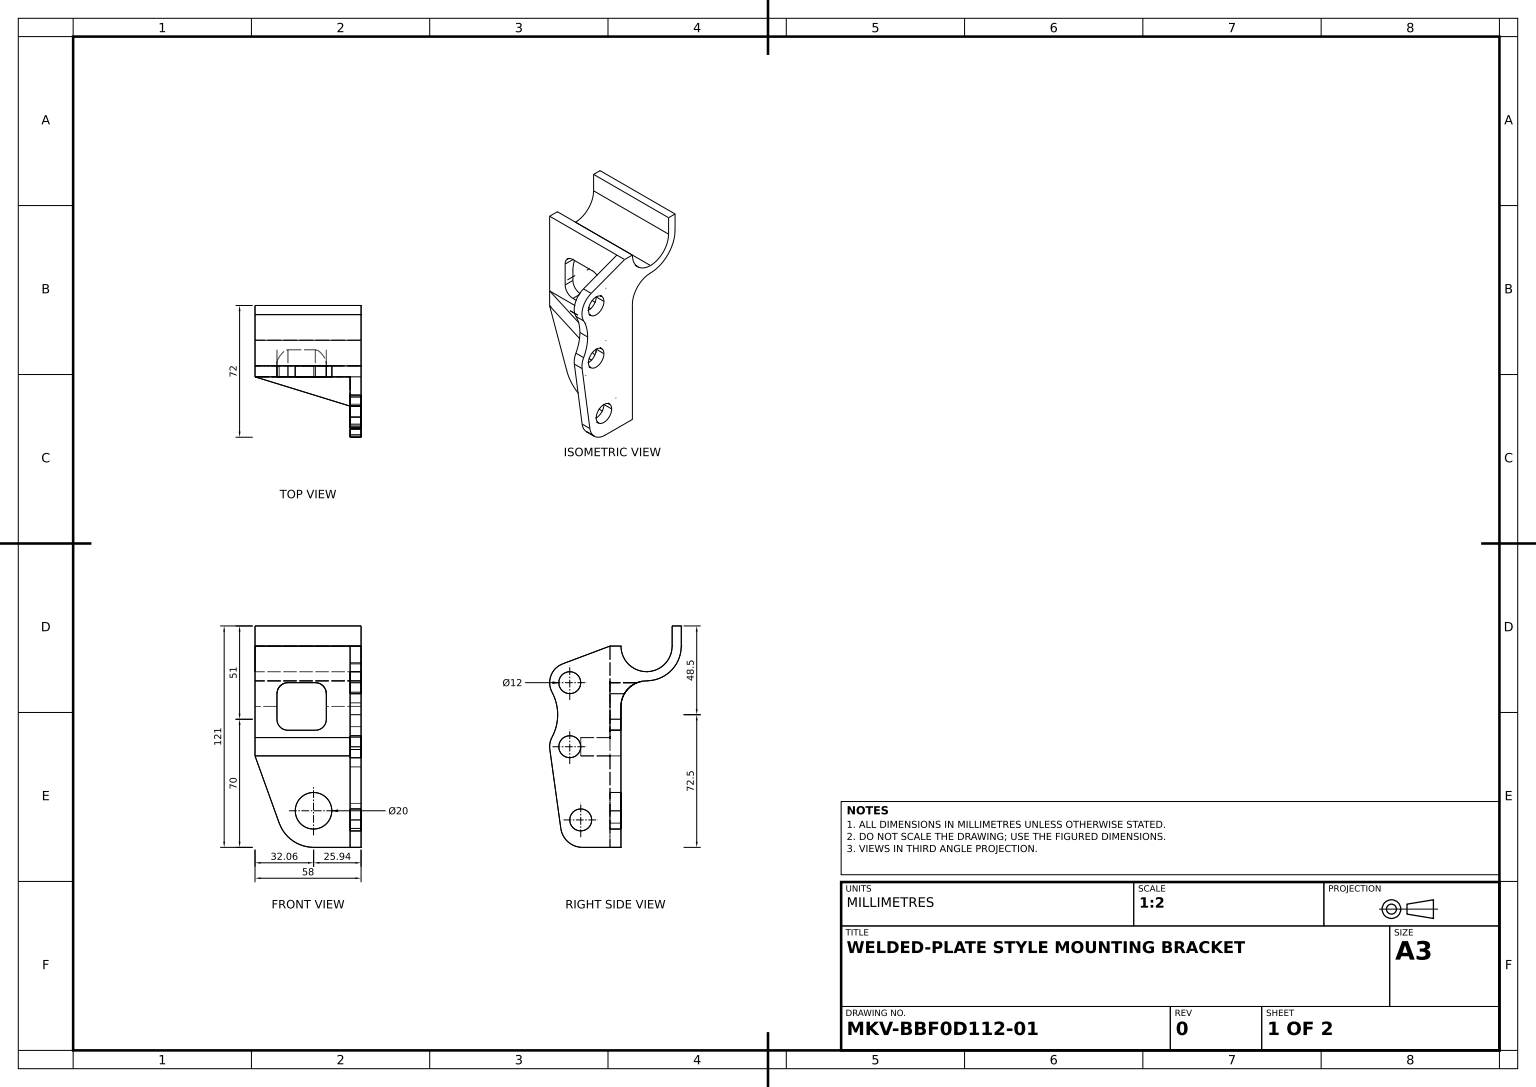
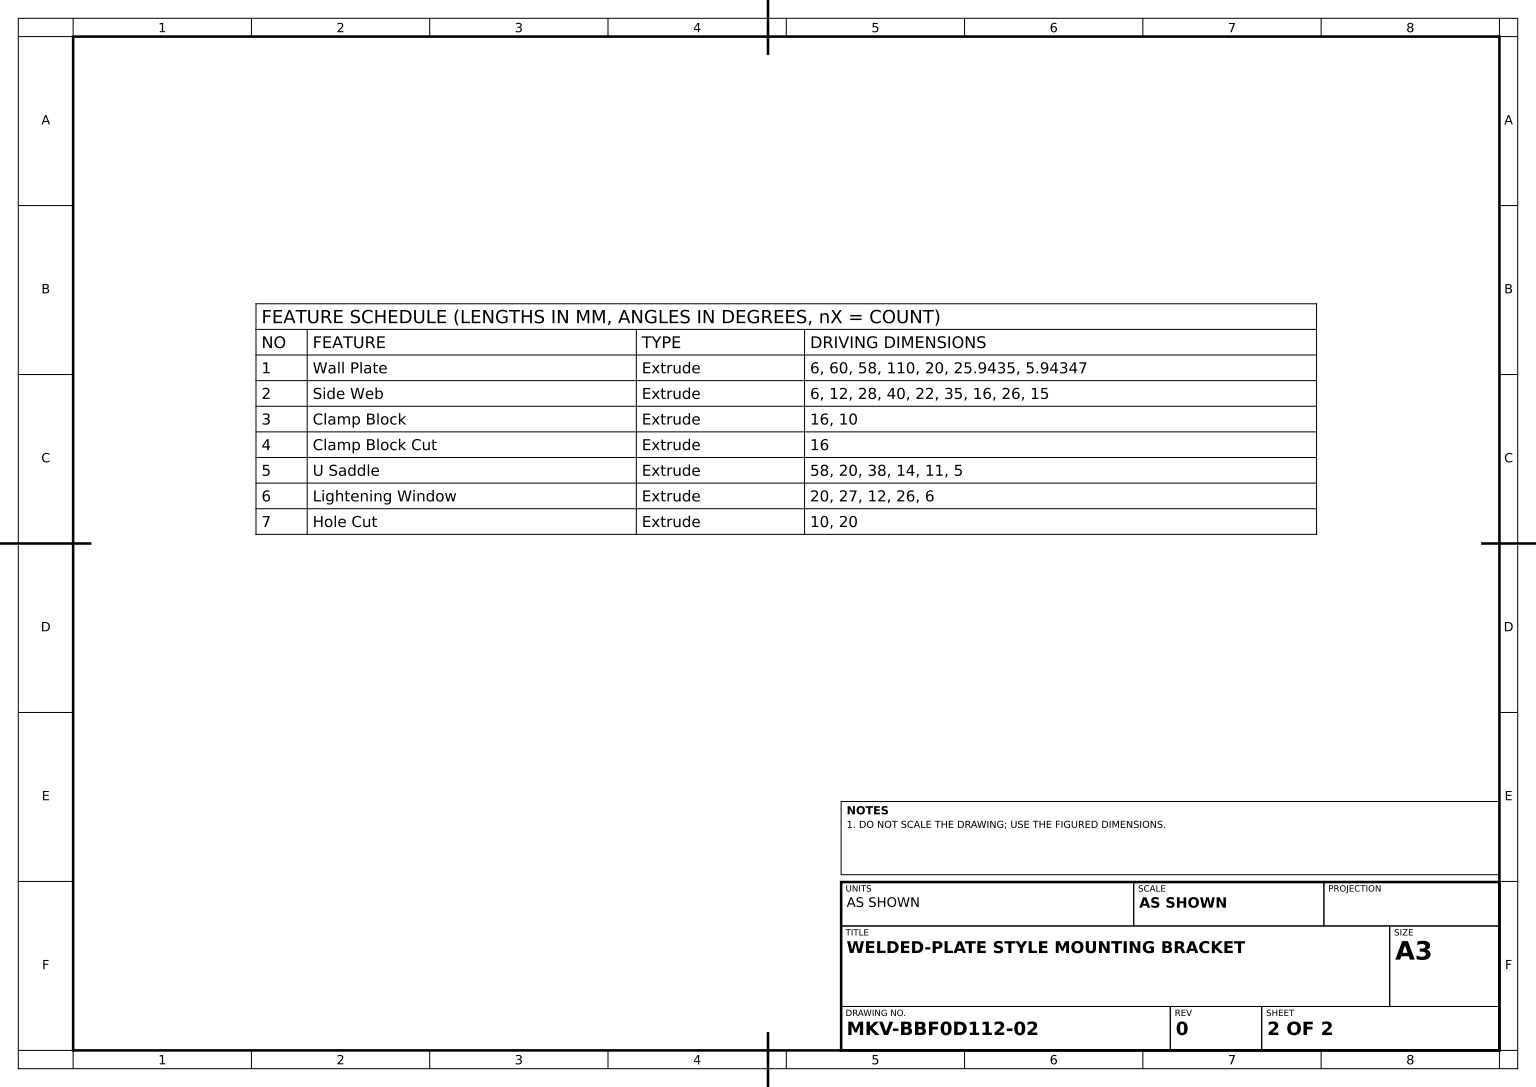
ISO-10303-21;
HEADER;
FILE_DESCRIPTION((''),'2;1');
FILE_NAME('','',(''),(''),'','','');
FILE_SCHEMA(('AUTOMOTIVE_DESIGN'));
ENDSEC;
DATA;
#1=APPLICATION_CONTEXT('');
#2=PRODUCT_CONTEXT('',#1,'mechanical');
#3=PRODUCT('','','',(#2));
#4=PRODUCT_DEFINITION_FORMATION('','',#3);
#5=PRODUCT_DEFINITION_CONTEXT('',#1,'design');
#6=PRODUCT_DEFINITION('','',#4,#5);
#7=PRODUCT_DEFINITION_SHAPE('','',#6);
#8=(LENGTH_UNIT()NAMED_UNIT(*)SI_UNIT(.MILLI.,.METRE.));
#9=(NAMED_UNIT(*)PLANE_ANGLE_UNIT()SI_UNIT($,.RADIAN.));
#10=(NAMED_UNIT(*)SI_UNIT($,.STERADIAN.)SOLID_ANGLE_UNIT());
#11=UNCERTAINTY_MEASURE_WITH_UNIT(LENGTH_MEASURE(1.E-05),#8,'distance_accuracy_value','');
#12=(GEOMETRIC_REPRESENTATION_CONTEXT(3)GLOBAL_UNCERTAINTY_ASSIGNED_CONTEXT((#11))GLOBAL_UNIT_ASSIGNED_CONTEXT((#8,#9,#10))REPRESENTATION_CONTEXT('',''));
#13=CARTESIAN_POINT('',(52.,0.,6.));
#14=VERTEX_POINT('',#13);
#15=CARTESIAN_POINT('',(0.,0.,6.));
#16=VERTEX_POINT('',#15);
#17=DIRECTION('',(-1.,0.,0.));
#18=VECTOR('',#17,1000.);
#19=LINE('',#15,#18);
#20=EDGE_CURVE('',#14,#16,#19,.T.);
#21=ORIENTED_EDGE('',*,*,#20,.F.);
#22=CARTESIAN_POINT('',(58.,0.,6.));
#23=VERTEX_POINT('',#22);
#24=EDGE_CURVE('',#23,#14,#19,.T.);
#25=ORIENTED_EDGE('',*,*,#24,.F.);
#26=CARTESIAN_POINT('',(58.,0.,0.));
#27=VERTEX_POINT('',#26);
#28=DIRECTION('',(0.,0.,-1.));
#29=VECTOR('',#28,1000.);
#30=LINE('',#22,#29);
#31=EDGE_CURVE('',#23,#27,#30,.T.);
#32=ORIENTED_EDGE('',*,*,#31,.T.);
#33=CARTESIAN_POINT('',(0.,0.,0.));
#34=VERTEX_POINT('',#33);
#35=LINE('',#33,#18);
#36=EDGE_CURVE('',#27,#34,#35,.T.);
#37=ORIENTED_EDGE('',*,*,#36,.T.);
#38=LINE('',#15,#29);
#39=EDGE_CURVE('',#16,#34,#38,.T.);
#40=ORIENTED_EDGE('',*,*,#39,.F.);
#41=EDGE_LOOP('',(#21,#25,#32,#37,#40));
#42=FACE_OUTER_BOUND('',#41,.T.);
#43=DIRECTION('',(0.,-1.,0.));
#44=AXIS2_PLACEMENT_3D('',#15,#43,#28);
#45=PLANE('',#44);
#46=ADVANCED_FACE('',(#42),#45,.F.);
#47=CARTESIAN_POINT('',(52.,-95.,16.));
#48=VERTEX_POINT('',#47);
#49=CARTESIAN_POINT('',(58.,-95.,16.));
#50=VERTEX_POINT('',#49);
#51=DIRECTION('',(1.,0.,0.));
#52=VECTOR('',#51,1000.);
#53=LINE('',#47,#52);
#54=EDGE_CURVE('',#48,#50,#53,.T.);
#55=ORIENTED_EDGE('',*,*,#54,.F.);
#56=CARTESIAN_POINT('',(52.,-95.,28.));
#57=VERTEX_POINT('',#56);
#58=CARTESIAN_POINT('',(52.,-95.,22.));
#59=AXIS2_PLACEMENT_3D('',#58,#51,#28);
#60=CIRCLE('',#59,6.);
#61=EDGE_CURVE('',#57,#48,#60,.T.);
#62=ORIENTED_EDGE('',*,*,#61,.F.);
#63=CARTESIAN_POINT('',(58.,-95.,28.));
#64=VERTEX_POINT('',#63);
#65=LINE('',#56,#52);
#66=EDGE_CURVE('',#57,#64,#65,.T.);
#67=ORIENTED_EDGE('',*,*,#66,.T.);
#68=CARTESIAN_POINT('',(58.,-95.,22.));
#69=AXIS2_PLACEMENT_3D('',#68,#51,#28);
#70=CIRCLE('',#69,6.);
#71=EDGE_CURVE('',#64,#50,#70,.T.);
#72=ORIENTED_EDGE('',*,*,#71,.T.);
#73=EDGE_LOOP('',(#55,#62,#67,#72));
#74=FACE_OUTER_BOUND('',#73,.T.);
#75=CYLINDRICAL_SURFACE('',#59,6.);
#76=ADVANCED_FACE('',(#74),#75,.F.);
#77=CARTESIAN_POINT('',(58.,11.,-33.));
#78=VERTEX_POINT('',#77);
#79=CARTESIAN_POINT('',(0.,11.,-33.));
#80=VERTEX_POINT('',#79);
#81=LINE('',#77,#18);
#82=EDGE_CURVE('',#78,#80,#81,.T.);
#83=ORIENTED_EDGE('',*,*,#82,.F.);
#84=CARTESIAN_POINT('',(58.,0.,-33.));
#85=VERTEX_POINT('',#84);
#86=DIRECTION('',(0.,1.,0.));
#87=VECTOR('',#86,1000.);
#88=LINE('',#84,#87);
#89=EDGE_CURVE('',#85,#78,#88,.T.);
#90=ORIENTED_EDGE('',*,*,#89,.F.);
#91=CARTESIAN_POINT('',(0.,0.,-33.));
#92=VERTEX_POINT('',#91);
#93=LINE('',#84,#18);
#94=EDGE_CURVE('',#85,#92,#93,.T.);
#95=ORIENTED_EDGE('',*,*,#94,.T.);
#96=LINE('',#91,#87);
#97=EDGE_CURVE('',#92,#80,#96,.T.);
#98=ORIENTED_EDGE('',*,*,#97,.T.);
#99=EDGE_LOOP('',(#83,#90,#95,#98));
#100=FACE_OUTER_BOUND('',#99,.T.);
#101=DIRECTION('',(0.,0.,1.));
#102=AXIS2_PLACEMENT_3D('',#84,#101,#51);
#103=PLANE('',#102);
#104=ADVANCED_FACE('',(#100),#103,.F.);
#105=CARTESIAN_POINT('',(22.,-90.,0.));
#106=VERTEX_POINT('',#105);
#107=CARTESIAN_POINT('',(22.,-90.,6.));
#108=VERTEX_POINT('',#107);
#109=CARTESIAN_POINT('',(22.,-90.,-4.));
#110=VECTOR('',#101,1000.);
#111=LINE('',#109,#110);
#112=EDGE_CURVE('',#106,#108,#111,.T.);
#113=ORIENTED_EDGE('',*,*,#112,.F.);
#114=CARTESIAN_POINT('',(42.,-90.,0.));
#115=VERTEX_POINT('',#114);
#116=CARTESIAN_POINT('',(32.,-90.,0.));
#117=AXIS2_PLACEMENT_3D('',#116,#28,#17);
#118=CIRCLE('',#117,10.);
#119=EDGE_CURVE('',#106,#115,#118,.T.);
#120=ORIENTED_EDGE('',*,*,#119,.T.);
#121=CARTESIAN_POINT('',(42.,-90.,6.));
#122=VERTEX_POINT('',#121);
#123=CARTESIAN_POINT('',(42.,-90.,-4.));
#124=LINE('',#123,#110);
#125=EDGE_CURVE('',#115,#122,#124,.T.);
#126=ORIENTED_EDGE('',*,*,#125,.T.);
#127=CARTESIAN_POINT('',(32.,-90.,6.));
#128=AXIS2_PLACEMENT_3D('',#127,#101,#51);
#129=CIRCLE('',#128,10.);
#130=EDGE_CURVE('',#122,#108,#129,.T.);
#131=ORIENTED_EDGE('',*,*,#130,.T.);
#132=EDGE_LOOP('',(#113,#120,#126,#131));
#133=FACE_OUTER_BOUND('',#132,.T.);
#134=CARTESIAN_POINT('',(32.,-90.,-4.));
#135=AXIS2_PLACEMENT_3D('',#134,#101,#51);
#136=CYLINDRICAL_SURFACE('',#135,10.);
#137=ADVANCED_FACE('',(#133),#136,.F.);
#138=EDGE_CURVE('',#48,#57,#60,.T.);
#139=ORIENTED_EDGE('',*,*,#138,.F.);
#140=ORIENTED_EDGE('',*,*,#54,.T.);
#141=EDGE_CURVE('',#50,#64,#70,.T.);
#142=ORIENTED_EDGE('',*,*,#141,.T.);
#143=ORIENTED_EDGE('',*,*,#66,.F.);
#144=EDGE_LOOP('',(#139,#140,#142,#143));
#145=FACE_OUTER_BOUND('',#144,.T.);
#146=ADVANCED_FACE('',(#145),#75,.F.);
#147=CARTESIAN_POINT('',(58.,-20.,22.));
#148=VERTEX_POINT('',#147);
#149=CARTESIAN_POINT('',(58.,-20.,34.));
#150=VERTEX_POINT('',#149);
#151=CARTESIAN_POINT('',(58.,-20.,28.));
#152=AXIS2_PLACEMENT_3D('',#151,#51,#28);
#153=CIRCLE('',#152,6.);
#154=EDGE_CURVE('',#148,#150,#153,.T.);
#155=ORIENTED_EDGE('',*,*,#154,.T.);
#156=CARTESIAN_POINT('',(52.,-20.,34.));
#157=VERTEX_POINT('',#156);
#158=LINE('',#156,#52);
#159=EDGE_CURVE('',#157,#150,#158,.T.);
#160=ORIENTED_EDGE('',*,*,#159,.F.);
#161=CARTESIAN_POINT('',(52.,-20.,22.));
#162=VERTEX_POINT('',#161);
#163=CARTESIAN_POINT('',(52.,-20.,28.));
#164=AXIS2_PLACEMENT_3D('',#163,#51,#28);
#165=CIRCLE('',#164,6.);
#166=EDGE_CURVE('',#162,#157,#165,.T.);
#167=ORIENTED_EDGE('',*,*,#166,.F.);
#168=LINE('',#161,#52);
#169=EDGE_CURVE('',#162,#148,#168,.T.);
#170=ORIENTED_EDGE('',*,*,#169,.T.);
#171=EDGE_LOOP('',(#155,#160,#167,#170));
#172=FACE_OUTER_BOUND('',#171,.T.);
#173=CYLINDRICAL_SURFACE('',#164,6.);
#174=ADVANCED_FACE('',(#172),#173,.F.);
#175=CARTESIAN_POINT('',(12.,-26.,-1.875644));
#176=VERTEX_POINT('',#175);
#177=CARTESIAN_POINT('',(12.,-26.,6.));
#178=VERTEX_POINT('',#177);
#179=CARTESIAN_POINT('',(12.,-26.,-14.));
#180=LINE('',#179,#110);
#181=EDGE_CURVE('',#176,#178,#180,.T.);
#182=ORIENTED_EDGE('',*,*,#181,.T.);
#183=CARTESIAN_POINT('',(12.,-40.,6.));
#184=VERTEX_POINT('',#183);
#185=VECTOR('',#43,1000.);
#186=LINE('',#177,#185);
#187=EDGE_CURVE('',#178,#184,#186,.T.);
#188=ORIENTED_EDGE('',*,*,#187,.T.);
#189=CARTESIAN_POINT('',(12.,-40.,0.));
#190=VERTEX_POINT('',#189);
#191=CARTESIAN_POINT('',(12.,-40.,-14.));
#192=LINE('',#191,#110);
#193=EDGE_CURVE('',#190,#184,#192,.T.);
#194=ORIENTED_EDGE('',*,*,#193,.F.);
#195=CARTESIAN_POINT('',(12.,-33.,0.));
#196=VERTEX_POINT('',#195);
#197=CARTESIAN_POINT('',(12.,-90.,0.));
#198=LINE('',#197,#87);
#199=EDGE_CURVE('',#190,#196,#198,.T.);
#200=ORIENTED_EDGE('',*,*,#199,.T.);
#201=CARTESIAN_POINT('',(12.,-33.,-14.));
#202=AXIS2_PLACEMENT_3D('',#201,#17,#101);
#203=CIRCLE('',#202,14.);
#204=EDGE_CURVE('',#196,#176,#203,.T.);
#205=ORIENTED_EDGE('',*,*,#204,.T.);
#206=EDGE_LOOP('',(#182,#188,#194,#200,#205));
#207=FACE_OUTER_BOUND('',#206,.T.);
#208=AXIS2_PLACEMENT_3D('',#179,#17,#101);
#209=PLANE('',#208);
#210=ADVANCED_FACE('',(#207),#209,.F.);
#211=EDGE_CURVE('',#115,#106,#118,.T.);
#212=ORIENTED_EDGE('',*,*,#211,.F.);
#213=ORIENTED_EDGE('',*,*,#119,.F.);
#214=EDGE_LOOP('',(#212,#213));
#215=FACE_BOUND('',#214,.T.);
#216=CARTESIAN_POINT('',(32.056528,-110.,0.));
#217=VERTEX_POINT('',#216);
#218=CARTESIAN_POINT('',(58.,-110.,0.));
#219=VERTEX_POINT('',#218);
#220=LINE('',#218,#52);
#221=EDGE_CURVE('',#217,#219,#220,.T.);
#222=ORIENTED_EDGE('',*,*,#221,.F.);
#223=CARTESIAN_POINT('',(13.23878,-96.774389,0.));
#224=VERTEX_POINT('',#223);
#225=CARTESIAN_POINT('',(32.056528,-90.,0.));
#226=AXIS2_PLACEMENT_3D('',#225,#101,#17);
#227=CIRCLE('',#226,20.);
#228=EDGE_CURVE('',#224,#217,#227,.T.);
#229=ORIENTED_EDGE('',*,*,#228,.F.);
#230=CARTESIAN_POINT('',(0.,-60.,0.));
#231=VERTEX_POINT('',#230);
#232=DIRECTION('',(0.338719468,-0.940887412,0.));
#233=VECTOR('',#232,1000.);
#234=LINE('',#223,#233);
#235=EDGE_CURVE('',#231,#224,#234,.T.);
#236=ORIENTED_EDGE('',*,*,#235,.F.);
#237=CARTESIAN_POINT('',(0.,-33.,0.));
#238=VERTEX_POINT('',#237);
#239=LINE('',#33,#185);
#240=EDGE_CURVE('',#238,#231,#239,.T.);
#241=ORIENTED_EDGE('',*,*,#240,.F.);
#242=CARTESIAN_POINT('',(58.,-33.,0.));
#243=LINE('',#242,#18);
#244=EDGE_CURVE('',#196,#238,#243,.T.);
#245=ORIENTED_EDGE('',*,*,#244,.F.);
#246=ORIENTED_EDGE('',*,*,#199,.F.);
#247=CARTESIAN_POINT('',(18.,-46.,0.));
#248=VERTEX_POINT('',#247);
#249=CARTESIAN_POINT('',(18.,-40.,0.));
#250=AXIS2_PLACEMENT_3D('',#249,#28,#17);
#251=CIRCLE('',#250,6.);
#252=EDGE_CURVE('',#248,#190,#251,.T.);
#253=ORIENTED_EDGE('',*,*,#252,.F.);
#254=CARTESIAN_POINT('',(33.,-46.,0.));
#255=VERTEX_POINT('',#254);
#256=CARTESIAN_POINT('',(32.056528,-46.,0.));
#257=LINE('',#256,#18);
#258=EDGE_CURVE('',#255,#248,#257,.T.);
#259=ORIENTED_EDGE('',*,*,#258,.F.);
#260=CARTESIAN_POINT('',(39.,-40.,0.));
#261=VERTEX_POINT('',#260);
#262=CARTESIAN_POINT('',(33.,-40.,0.));
#263=AXIS2_PLACEMENT_3D('',#262,#28,#17);
#264=CIRCLE('',#263,6.);
#265=EDGE_CURVE('',#261,#255,#264,.T.);
#266=ORIENTED_EDGE('',*,*,#265,.F.);
#267=CARTESIAN_POINT('',(39.,-33.,0.));
#268=VERTEX_POINT('',#267);
#269=CARTESIAN_POINT('',(39.,-90.,0.));
#270=LINE('',#269,#185);
#271=EDGE_CURVE('',#268,#261,#270,.T.);
#272=ORIENTED_EDGE('',*,*,#271,.F.);
#273=VERTEX_POINT('',#242);
#274=EDGE_CURVE('',#273,#268,#243,.T.);
#275=ORIENTED_EDGE('',*,*,#274,.F.);
#276=LINE('',#26,#87);
#277=EDGE_CURVE('',#219,#273,#276,.T.);
#278=ORIENTED_EDGE('',*,*,#277,.F.);
#279=EDGE_LOOP('',(#222,#229,#236,#241,#245,#246,#253,#259,#266,#272,#275,#278));
#280=FACE_OUTER_BOUND('',#279,.T.);
#281=AXIS2_PLACEMENT_3D('',#225,#28,#17);
#282=PLANE('',#281);
#283=ADVANCED_FACE('',(#215,#280),#282,.T.);
#284=CARTESIAN_POINT('',(0.,-60.,6.));
#285=VERTEX_POINT('',#284);
#286=CARTESIAN_POINT('',(52.,-60.,6.));
#287=VERTEX_POINT('',#286);
#288=LINE('',#284,#52);
#289=EDGE_CURVE('',#285,#287,#288,.T.);
#290=ORIENTED_EDGE('',*,*,#289,.T.);
#291=CARTESIAN_POINT('',(52.,-60.,22.));
#292=VERTEX_POINT('',#291);
#293=LINE('',#291,#29);
#294=EDGE_CURVE('',#292,#287,#293,.T.);
#295=ORIENTED_EDGE('',*,*,#294,.F.);
#296=CARTESIAN_POINT('',(4.497297,-60.,7.383784));
#297=DIRECTION('',(0.955779009,0.,0.294085849));
#298=VECTOR('',#297,1000.);
#299=LINE('',#296,#298);
#300=EDGE_CURVE('',#285,#292,#299,.T.);
#301=ORIENTED_EDGE('',*,*,#300,.F.);
#302=EDGE_LOOP('',(#290,#295,#301));
#303=FACE_OUTER_BOUND('',#302,.T.);
#304=CARTESIAN_POINT('',(0.,-60.,22.));
#305=AXIS2_PLACEMENT_3D('',#304,#86,#101);
#306=PLANE('',#305);
#307=ADVANCED_FACE('',(#303),#306,.F.);
#308=CARTESIAN_POINT('',(52.,-25.202703,37.691846));
#309=VERTEX_POINT('',#308);
#310=CARTESIAN_POINT('',(52.,-37.5,34.599847));
#311=VERTEX_POINT('',#310);
#312=CARTESIAN_POINT('',(52.,-37.5,60.599847));
#313=AXIS2_PLACEMENT_3D('',#312,#17,#28);
#314=CIRCLE('',#313,26.);
#315=EDGE_CURVE('',#309,#311,#314,.T.);
#316=ORIENTED_EDGE('',*,*,#315,.T.);
#317=CARTESIAN_POINT('',(58.,-37.5,34.599847));
#318=VERTEX_POINT('',#317);
#319=LINE('',#310,#52);
#320=EDGE_CURVE('',#311,#318,#319,.T.);
#321=ORIENTED_EDGE('',*,*,#320,.T.);
#322=CARTESIAN_POINT('',(58.,-25.202703,37.691846));
#323=VERTEX_POINT('',#322);
#324=CARTESIAN_POINT('',(58.,-37.5,60.599847));
#325=AXIS2_PLACEMENT_3D('',#324,#17,#28);
#326=CIRCLE('',#325,26.);
#327=EDGE_CURVE('',#323,#318,#326,.T.);
#328=ORIENTED_EDGE('',*,*,#327,.F.);
#329=LINE('',#308,#52);
#330=EDGE_CURVE('',#309,#323,#329,.T.);
#331=ORIENTED_EDGE('',*,*,#330,.F.);
#332=EDGE_LOOP('',(#316,#321,#328,#331));
#333=FACE_OUTER_BOUND('',#332,.T.);
#334=AXIS2_PLACEMENT_3D('',#312,#51,#28);
#335=CYLINDRICAL_SURFACE('',#334,26.);
#336=ADVANCED_FACE('',(#333),#335,.F.);
#337=CARTESIAN_POINT('',(52.,-110.,6.));
#338=VERTEX_POINT('',#337);
#339=CARTESIAN_POINT('',(52.,-110.,21.));
#340=VERTEX_POINT('',#339);
#341=CARTESIAN_POINT('',(52.,-110.,0.));
#342=LINE('',#341,#110);
#343=EDGE_CURVE('',#338,#340,#342,.T.);
#344=ORIENTED_EDGE('',*,*,#343,.F.);
#345=CARTESIAN_POINT('',(32.056528,-110.,6.));
#346=VERTEX_POINT('',#345);
#347=CARTESIAN_POINT('',(38.,-110.,6.));
#348=LINE('',#347,#52);
#349=EDGE_CURVE('',#346,#338,#348,.T.);
#350=ORIENTED_EDGE('',*,*,#349,.F.);
#351=LINE('',#345,#29);
#352=EDGE_CURVE('',#346,#217,#351,.T.);
#353=ORIENTED_EDGE('',*,*,#352,.T.);
#354=ORIENTED_EDGE('',*,*,#221,.T.);
#355=CARTESIAN_POINT('',(58.,-110.,21.));
#356=VERTEX_POINT('',#355);
#357=CARTESIAN_POINT('',(58.,-110.,6.));
#358=LINE('',#357,#29);
#359=EDGE_CURVE('',#356,#219,#358,.T.);
#360=ORIENTED_EDGE('',*,*,#359,.F.);
#361=LINE('',#339,#52);
#362=EDGE_CURVE('',#340,#356,#361,.T.);
#363=ORIENTED_EDGE('',*,*,#362,.F.);
#364=EDGE_LOOP('',(#344,#350,#353,#354,#360,#363));
#365=FACE_OUTER_BOUND('',#364,.T.);
#366=AXIS2_PLACEMENT_3D('',#357,#86,#101);
#367=PLANE('',#366);
#368=ADVANCED_FACE('',(#365),#367,.F.);
#369=CARTESIAN_POINT('',(52.,-9.70064,31.863054));
#370=VERTEX_POINT('',#369);
#371=CIRCLE('',#164,11.);
#372=EDGE_CURVE('',#370,#309,#371,.T.);
#373=ORIENTED_EDGE('',*,*,#372,.T.);
#374=ORIENTED_EDGE('',*,*,#330,.T.);
#375=CARTESIAN_POINT('',(58.,-9.70064,31.863054));
#376=VERTEX_POINT('',#375);
#377=CIRCLE('',#152,11.);
#378=EDGE_CURVE('',#376,#323,#377,.T.);
#379=ORIENTED_EDGE('',*,*,#378,.F.);
#380=LINE('',#369,#52);
#381=EDGE_CURVE('',#370,#376,#380,.T.);
#382=ORIENTED_EDGE('',*,*,#381,.F.);
#383=EDGE_LOOP('',(#373,#374,#379,#382));
#384=FACE_OUTER_BOUND('',#383,.T.);
#385=CYLINDRICAL_SURFACE('',#164,11.);
#386=ADVANCED_FACE('',(#384),#385,.T.);
#387=CARTESIAN_POINT('',(52.,-50.,6.));
#388=VERTEX_POINT('',#387);
#389=CARTESIAN_POINT('',(0.,-50.,6.));
#390=VERTEX_POINT('',#389);
#391=LINE('',#389,#18);
#392=EDGE_CURVE('',#388,#390,#391,.T.);
#393=ORIENTED_EDGE('',*,*,#392,.T.);
#394=CARTESIAN_POINT('',(52.,-50.,22.));
#395=VERTEX_POINT('',#394);
#396=LINE('',#394,#298);
#397=EDGE_CURVE('',#390,#395,#396,.T.);
#398=ORIENTED_EDGE('',*,*,#397,.T.);
#399=LINE('',#394,#29);
#400=EDGE_CURVE('',#395,#388,#399,.T.);
#401=ORIENTED_EDGE('',*,*,#400,.T.);
#402=EDGE_LOOP('',(#393,#398,#401));
#403=FACE_OUTER_BOUND('',#402,.T.);
#404=CARTESIAN_POINT('',(0.,-50.,22.));
#405=AXIS2_PLACEMENT_3D('',#404,#43,#28);
#406=PLANE('',#405);
#407=ADVANCED_FACE('',(#403),#406,.F.);
#408=CARTESIAN_POINT('',(52.,1.972908,0.739993));
#409=DIRECTION('',(0.,-0.351186756,0.936305432));
#410=VECTOR('',#409,1000.);
#411=LINE('',#408,#410);
#412=EDGE_CURVE('',#14,#370,#411,.T.);
#413=ORIENTED_EDGE('',*,*,#412,.T.);
#414=ORIENTED_EDGE('',*,*,#381,.T.);
#415=CARTESIAN_POINT('',(58.,1.972908,0.739993));
#416=LINE('',#415,#410);
#417=EDGE_CURVE('',#23,#376,#416,.T.);
#418=ORIENTED_EDGE('',*,*,#417,.F.);
#419=ORIENTED_EDGE('',*,*,#24,.T.);
#420=EDGE_LOOP('',(#413,#414,#418,#419));
#421=FACE_OUTER_BOUND('',#420,.T.);
#422=DIRECTION('',(0.,0.936305432,0.351186756));
#423=AXIS2_PLACEMENT_3D('',#408,#422,#409);
#424=PLANE('',#423);
#425=ADVANCED_FACE('',(#421),#424,.T.);
#426=CARTESIAN_POINT('',(58.,0.,-28.));
#427=VERTEX_POINT('',#426);
#428=CARTESIAN_POINT('',(0.,0.,-28.));
#429=VERTEX_POINT('',#428);
#430=LINE('',#426,#18);
#431=EDGE_CURVE('',#427,#429,#430,.T.);
#432=ORIENTED_EDGE('',*,*,#431,.F.);
#433=CARTESIAN_POINT('',(58.,11.,-28.));
#434=VERTEX_POINT('',#433);
#435=LINE('',#426,#87);
#436=EDGE_CURVE('',#427,#434,#435,.T.);
#437=ORIENTED_EDGE('',*,*,#436,.T.);
#438=CARTESIAN_POINT('',(0.,11.,-28.));
#439=VERTEX_POINT('',#438);
#440=LINE('',#433,#18);
#441=EDGE_CURVE('',#434,#439,#440,.T.);
#442=ORIENTED_EDGE('',*,*,#441,.T.);
#443=LINE('',#428,#87);
#444=EDGE_CURVE('',#429,#439,#443,.T.);
#445=ORIENTED_EDGE('',*,*,#444,.F.);
#446=EDGE_LOOP('',(#432,#437,#442,#445));
#447=FACE_OUTER_BOUND('',#446,.T.);
#448=AXIS2_PLACEMENT_3D('',#426,#101,#51);
#449=PLANE('',#448);
#450=ADVANCED_FACE('',(#447),#449,.T.);
#451=ORIENTED_EDGE('',*,*,#417,.T.);
#452=ORIENTED_EDGE('',*,*,#378,.T.);
#453=ORIENTED_EDGE('',*,*,#327,.T.);
#454=CARTESIAN_POINT('',(58.,-49.797297,37.691846));
#455=VERTEX_POINT('',#454);
#456=EDGE_CURVE('',#318,#455,#326,.T.);
#457=ORIENTED_EDGE('',*,*,#456,.T.);
#458=CARTESIAN_POINT('',(58.,-56.517756,38.894788));
#459=VERTEX_POINT('',#458);
#460=CARTESIAN_POINT('',(58.,-55.,28.));
#461=AXIS2_PLACEMENT_3D('',#460,#51,#28);
#462=CIRCLE('',#461,11.);
#463=EDGE_CURVE('',#455,#459,#462,.T.);
#464=ORIENTED_EDGE('',*,*,#463,.T.);
#465=CARTESIAN_POINT('',(58.,-99.655734,32.885224));
#466=VERTEX_POINT('',#465);
#467=CARTESIAN_POINT('',(58.,-6.391268,45.877925));
#468=DIRECTION('',(0.,0.990435316,0.137977842));
#469=VECTOR('',#468,1000.);
#470=LINE('',#467,#469);
#471=EDGE_CURVE('',#466,#459,#470,.T.);
#472=ORIENTED_EDGE('',*,*,#471,.F.);
#473=CARTESIAN_POINT('',(58.,-98.,21.));
#474=AXIS2_PLACEMENT_3D('',#473,#17,#28);
#475=CIRCLE('',#474,12.);
#476=EDGE_CURVE('',#356,#466,#475,.T.);
#477=ORIENTED_EDGE('',*,*,#476,.F.);
#478=ORIENTED_EDGE('',*,*,#359,.T.);
#479=ORIENTED_EDGE('',*,*,#277,.T.);
#480=CARTESIAN_POINT('',(58.,-19.,-14.));
#481=VERTEX_POINT('',#480);
#482=CARTESIAN_POINT('',(58.,-33.,-14.));
#483=AXIS2_PLACEMENT_3D('',#482,#51,#43);
#484=CIRCLE('',#483,14.);
#485=EDGE_CURVE('',#481,#273,#484,.T.);
#486=ORIENTED_EDGE('',*,*,#485,.F.);
#487=CARTESIAN_POINT('',(58.,0.,-14.));
#488=AXIS2_PLACEMENT_3D('',#487,#17,#43);
#489=CIRCLE('',#488,19.);
#490=EDGE_CURVE('',#85,#481,#489,.T.);
#491=ORIENTED_EDGE('',*,*,#490,.F.);
#492=ORIENTED_EDGE('',*,*,#89,.T.);
#493=CARTESIAN_POINT('',(58.,11.,0.));
#494=LINE('',#493,#29);
#495=EDGE_CURVE('',#434,#78,#494,.T.);
#496=ORIENTED_EDGE('',*,*,#495,.F.);
#497=ORIENTED_EDGE('',*,*,#436,.F.);
#498=CARTESIAN_POINT('',(58.,-14.,-14.));
#499=VERTEX_POINT('',#498);
#500=CIRCLE('',#488,14.);
#501=EDGE_CURVE('',#427,#499,#500,.T.);
#502=ORIENTED_EDGE('',*,*,#501,.T.);
#503=EDGE_CURVE('',#499,#27,#500,.T.);
#504=ORIENTED_EDGE('',*,*,#503,.T.);
#505=ORIENTED_EDGE('',*,*,#31,.F.);
#506=EDGE_LOOP('',(#451,#452,#453,#457,#464,#472,#477,#478,#479,#486,#491,#492,#496,#497,#502,#504,#505));
#507=FACE_OUTER_BOUND('',#506,.T.);
#508=ORIENTED_EDGE('',*,*,#154,.F.);
#509=EDGE_CURVE('',#150,#148,#153,.T.);
#510=ORIENTED_EDGE('',*,*,#509,.F.);
#511=EDGE_LOOP('',(#508,#510));
#512=FACE_BOUND('',#511,.T.);
#513=ORIENTED_EDGE('',*,*,#141,.F.);
#514=ORIENTED_EDGE('',*,*,#71,.F.);
#515=EDGE_LOOP('',(#513,#514));
#516=FACE_BOUND('',#515,.T.);
#517=CARTESIAN_POINT('',(58.,-55.,22.));
#518=VERTEX_POINT('',#517);
#519=CARTESIAN_POINT('',(58.,-55.,34.));
#520=VERTEX_POINT('',#519);
#521=CIRCLE('',#461,6.);
#522=EDGE_CURVE('',#518,#520,#521,.T.);
#523=ORIENTED_EDGE('',*,*,#522,.F.);
#524=EDGE_CURVE('',#520,#518,#521,.T.);
#525=ORIENTED_EDGE('',*,*,#524,.F.);
#526=EDGE_LOOP('',(#523,#525));
#527=FACE_BOUND('',#526,.T.);
#528=AXIS2_PLACEMENT_3D('',#22,#17,#101);
#529=PLANE('',#528);
#530=ADVANCED_FACE('',(#507,#512,#516,#527),#529,.F.);
#531=CARTESIAN_POINT('',(52.,-49.797297,37.691846));
#532=VERTEX_POINT('',#531);
#533=LINE('',#531,#52);
#534=EDGE_CURVE('',#532,#455,#533,.T.);
#535=ORIENTED_EDGE('',*,*,#534,.T.);
#536=ORIENTED_EDGE('',*,*,#456,.F.);
#537=ORIENTED_EDGE('',*,*,#320,.F.);
#538=EDGE_CURVE('',#311,#532,#314,.T.);
#539=ORIENTED_EDGE('',*,*,#538,.T.);
#540=EDGE_LOOP('',(#535,#536,#537,#539));
#541=FACE_OUTER_BOUND('',#540,.T.);
#542=ADVANCED_FACE('',(#541),#335,.F.);
#543=CARTESIAN_POINT('',(0.,-19.,-14.));
#544=VERTEX_POINT('',#543);
#545=LINE('',#480,#18);
#546=EDGE_CURVE('',#481,#544,#545,.T.);
#547=ORIENTED_EDGE('',*,*,#546,.T.);
#548=CARTESIAN_POINT('',(0.,0.,-14.));
#549=AXIS2_PLACEMENT_3D('',#548,#17,#43);
#550=CIRCLE('',#549,19.);
#551=EDGE_CURVE('',#92,#544,#550,.T.);
#552=ORIENTED_EDGE('',*,*,#551,.F.);
#553=ORIENTED_EDGE('',*,*,#94,.F.);
#554=ORIENTED_EDGE('',*,*,#490,.T.);
#555=EDGE_LOOP('',(#547,#552,#553,#554));
#556=FACE_OUTER_BOUND('',#555,.T.);
#557=CYLINDRICAL_SURFACE('',#488,19.);
#558=ADVANCED_FACE('',(#556),#557,.T.);
#559=ORIENTED_EDGE('',*,*,#503,.F.);
#560=CARTESIAN_POINT('',(0.,-14.,-14.));
#561=VERTEX_POINT('',#560);
#562=LINE('',#498,#18);
#563=EDGE_CURVE('',#499,#561,#562,.T.);
#564=ORIENTED_EDGE('',*,*,#563,.T.);
#565=CIRCLE('',#549,14.);
#566=EDGE_CURVE('',#561,#34,#565,.T.);
#567=ORIENTED_EDGE('',*,*,#566,.T.);
#568=ORIENTED_EDGE('',*,*,#36,.F.);
#569=EDGE_LOOP('',(#559,#564,#567,#568));
#570=FACE_OUTER_BOUND('',#569,.T.);
#571=CYLINDRICAL_SURFACE('',#488,14.);
#572=ADVANCED_FACE('',(#570),#571,.F.);
#573=ORIENTED_EDGE('',*,*,#125,.F.);
#574=ORIENTED_EDGE('',*,*,#211,.T.);
#575=ORIENTED_EDGE('',*,*,#112,.T.);
#576=EDGE_CURVE('',#108,#122,#129,.T.);
#577=ORIENTED_EDGE('',*,*,#576,.T.);
#578=EDGE_LOOP('',(#573,#574,#575,#577));
#579=FACE_OUTER_BOUND('',#578,.T.);
#580=ADVANCED_FACE('',(#579),#136,.F.);
#581=CARTESIAN_POINT('',(18.,-46.,6.));
#582=VERTEX_POINT('',#581);
#583=CARTESIAN_POINT('',(33.,-46.,6.));
#584=VERTEX_POINT('',#583);
#585=LINE('',#581,#52);
#586=EDGE_CURVE('',#582,#584,#585,.T.);
#587=ORIENTED_EDGE('',*,*,#586,.F.);
#588=CARTESIAN_POINT('',(18.,-40.,6.));
#589=AXIS2_PLACEMENT_3D('',#588,#101,#51);
#590=CIRCLE('',#589,6.);
#591=EDGE_CURVE('',#184,#582,#590,.T.);
#592=ORIENTED_EDGE('',*,*,#591,.F.);
#593=ORIENTED_EDGE('',*,*,#187,.F.);
#594=CARTESIAN_POINT('',(18.,-20.,6.));
#595=VERTEX_POINT('',#594);
#596=CARTESIAN_POINT('',(18.,-26.,6.));
#597=AXIS2_PLACEMENT_3D('',#596,#101,#51);
#598=CIRCLE('',#597,6.);
#599=EDGE_CURVE('',#595,#178,#598,.T.);
#600=ORIENTED_EDGE('',*,*,#599,.F.);
#601=CARTESIAN_POINT('',(33.,-20.,6.));
#602=VERTEX_POINT('',#601);
#603=LINE('',#594,#18);
#604=EDGE_CURVE('',#602,#595,#603,.T.);
#605=ORIENTED_EDGE('',*,*,#604,.F.);
#606=CARTESIAN_POINT('',(39.,-26.,6.));
#607=VERTEX_POINT('',#606);
#608=CARTESIAN_POINT('',(33.,-26.,6.));
#609=AXIS2_PLACEMENT_3D('',#608,#101,#17);
#610=CIRCLE('',#609,6.);
#611=EDGE_CURVE('',#607,#602,#610,.T.);
#612=ORIENTED_EDGE('',*,*,#611,.F.);
#613=CARTESIAN_POINT('',(39.,-40.,6.));
#614=VERTEX_POINT('',#613);
#615=LINE('',#606,#87);
#616=EDGE_CURVE('',#614,#607,#615,.T.);
#617=ORIENTED_EDGE('',*,*,#616,.F.);
#618=CARTESIAN_POINT('',(33.,-40.,6.));
#619=AXIS2_PLACEMENT_3D('',#618,#101,#51);
#620=CIRCLE('',#619,6.);
#621=EDGE_CURVE('',#584,#614,#620,.T.);
#622=ORIENTED_EDGE('',*,*,#621,.F.);
#623=EDGE_LOOP('',(#587,#592,#593,#600,#605,#612,#617,#622));
#624=FACE_BOUND('',#623,.T.);
#625=LINE('',#13,#185);
#626=EDGE_CURVE('',#14,#388,#625,.T.);
#627=ORIENTED_EDGE('',*,*,#626,.F.);
#628=ORIENTED_EDGE('',*,*,#20,.T.);
#629=LINE('',#15,#185);
#630=EDGE_CURVE('',#16,#390,#629,.T.);
#631=ORIENTED_EDGE('',*,*,#630,.T.);
#632=ORIENTED_EDGE('',*,*,#392,.F.);
#633=EDGE_LOOP('',(#627,#628,#631,#632));
#634=FACE_OUTER_BOUND('',#633,.T.);
#635=CARTESIAN_POINT('',(32.056528,-90.,6.));
#636=AXIS2_PLACEMENT_3D('',#635,#28,#17);
#637=PLANE('',#636);
#638=ADVANCED_FACE('',(#624,#634),#637,.F.);
#639=ORIENTED_EDGE('',*,*,#431,.T.);
#640=EDGE_CURVE('',#429,#561,#565,.T.);
#641=ORIENTED_EDGE('',*,*,#640,.T.);
#642=ORIENTED_EDGE('',*,*,#563,.F.);
#643=ORIENTED_EDGE('',*,*,#501,.F.);
#644=EDGE_LOOP('',(#639,#641,#642,#643));
#645=FACE_OUTER_BOUND('',#644,.T.);
#646=ADVANCED_FACE('',(#645),#571,.F.);
#647=CARTESIAN_POINT('',(52.,-56.517756,38.894788));
#648=VERTEX_POINT('',#647);
#649=CARTESIAN_POINT('',(52.,-55.,28.));
#650=AXIS2_PLACEMENT_3D('',#649,#51,#28);
#651=CIRCLE('',#650,11.);
#652=EDGE_CURVE('',#532,#648,#651,.T.);
#653=ORIENTED_EDGE('',*,*,#652,.T.);
#654=LINE('',#647,#52);
#655=EDGE_CURVE('',#648,#459,#654,.T.);
#656=ORIENTED_EDGE('',*,*,#655,.T.);
#657=ORIENTED_EDGE('',*,*,#463,.F.);
#658=ORIENTED_EDGE('',*,*,#534,.F.);
#659=EDGE_LOOP('',(#653,#656,#657,#658));
#660=FACE_OUTER_BOUND('',#659,.T.);
#661=CYLINDRICAL_SURFACE('',#650,11.);
#662=ADVANCED_FACE('',(#660),#661,.T.);
#663=ORIENTED_EDGE('',*,*,#265,.T.);
#664=CARTESIAN_POINT('',(33.,-46.,-14.));
#665=LINE('',#664,#110);
#666=EDGE_CURVE('',#255,#584,#665,.T.);
#667=ORIENTED_EDGE('',*,*,#666,.T.);
#668=ORIENTED_EDGE('',*,*,#621,.T.);
#669=CARTESIAN_POINT('',(39.,-40.,-14.));
#670=LINE('',#669,#110);
#671=EDGE_CURVE('',#261,#614,#670,.T.);
#672=ORIENTED_EDGE('',*,*,#671,.F.);
#673=EDGE_LOOP('',(#663,#667,#668,#672));
#674=FACE_OUTER_BOUND('',#673,.T.);
#675=CARTESIAN_POINT('',(33.,-40.,-14.));
#676=AXIS2_PLACEMENT_3D('',#675,#101,#51);
#677=CYLINDRICAL_SURFACE('',#676,6.);
#678=ADVANCED_FACE('',(#674),#677,.F.);
#679=CARTESIAN_POINT('',(18.,-20.,-8.803848));
#680=VERTEX_POINT('',#679);
#681=CARTESIAN_POINT('',(18.,-20.,-14.));
#682=LINE('',#681,#110);
#683=EDGE_CURVE('',#680,#595,#682,.T.);
#684=ORIENTED_EDGE('',*,*,#683,.F.);
#685=CARTESIAN_POINT('',(33.,-20.,-8.803848));
#686=VERTEX_POINT('',#685);
#687=CARTESIAN_POINT('',(58.,-20.,-8.803848));
#688=LINE('',#687,#52);
#689=EDGE_CURVE('',#680,#686,#688,.T.);
#690=ORIENTED_EDGE('',*,*,#689,.T.);
#691=CARTESIAN_POINT('',(33.,-20.,-14.));
#692=LINE('',#691,#110);
#693=EDGE_CURVE('',#686,#602,#692,.T.);
#694=ORIENTED_EDGE('',*,*,#693,.T.);
#695=ORIENTED_EDGE('',*,*,#604,.T.);
#696=EDGE_LOOP('',(#684,#690,#694,#695));
#697=FACE_OUTER_BOUND('',#696,.T.);
#698=AXIS2_PLACEMENT_3D('',#681,#86,#17);
#699=PLANE('',#698);
#700=ADVANCED_FACE('',(#697),#699,.F.);
#701=CARTESIAN_POINT('',(13.23878,-96.774389,6.));
#702=VERTEX_POINT('',#701);
#703=LINE('',#701,#233);
#704=EDGE_CURVE('',#285,#702,#703,.T.);
#705=ORIENTED_EDGE('',*,*,#704,.F.);
#706=LINE('',#284,#29);
#707=EDGE_CURVE('',#285,#231,#706,.T.);
#708=ORIENTED_EDGE('',*,*,#707,.T.);
#709=ORIENTED_EDGE('',*,*,#235,.T.);
#710=LINE('',#701,#29);
#711=EDGE_CURVE('',#702,#224,#710,.T.);
#712=ORIENTED_EDGE('',*,*,#711,.F.);
#713=EDGE_LOOP('',(#705,#708,#709,#712));
#714=FACE_OUTER_BOUND('',#713,.T.);
#715=DIRECTION('',(0.940887412,0.338719468,0.));
#716=DIRECTION('',(-0.338719468,0.940887412,0.));
#717=AXIS2_PLACEMENT_3D('',#701,#715,#716);
#718=PLANE('',#717);
#719=ADVANCED_FACE('',(#714),#718,.F.);
#720=CARTESIAN_POINT('',(18.,-46.,-14.));
#721=LINE('',#720,#110);
#722=EDGE_CURVE('',#248,#582,#721,.T.);
#723=ORIENTED_EDGE('',*,*,#722,.T.);
#724=ORIENTED_EDGE('',*,*,#586,.T.);
#725=ORIENTED_EDGE('',*,*,#666,.F.);
#726=ORIENTED_EDGE('',*,*,#258,.T.);
#727=EDGE_LOOP('',(#723,#724,#725,#726));
#728=FACE_OUTER_BOUND('',#727,.T.);
#729=AXIS2_PLACEMENT_3D('',#720,#43,#51);
#730=PLANE('',#729);
#731=ADVANCED_FACE('',(#728),#730,.F.);
#732=CARTESIAN_POINT('',(52.,-55.,34.));
#733=VERTEX_POINT('',#732);
#734=LINE('',#732,#52);
#735=EDGE_CURVE('',#733,#520,#734,.T.);
#736=ORIENTED_EDGE('',*,*,#735,.F.);
#737=CARTESIAN_POINT('',(52.,-55.,22.));
#738=VERTEX_POINT('',#737);
#739=CIRCLE('',#650,6.);
#740=EDGE_CURVE('',#738,#733,#739,.T.);
#741=ORIENTED_EDGE('',*,*,#740,.F.);
#742=LINE('',#737,#52);
#743=EDGE_CURVE('',#738,#518,#742,.T.);
#744=ORIENTED_EDGE('',*,*,#743,.T.);
#745=ORIENTED_EDGE('',*,*,#522,.T.);
#746=EDGE_LOOP('',(#736,#741,#744,#745));
#747=FACE_OUTER_BOUND('',#746,.T.);
#748=CYLINDRICAL_SURFACE('',#650,6.);
#749=ADVANCED_FACE('',(#747),#748,.F.);
#750=ORIENTED_EDGE('',*,*,#244,.T.);
#751=CARTESIAN_POINT('',(0.,-33.,-14.));
#752=AXIS2_PLACEMENT_3D('',#751,#51,#43);
#753=CIRCLE('',#752,14.);
#754=EDGE_CURVE('',#544,#238,#753,.T.);
#755=ORIENTED_EDGE('',*,*,#754,.F.);
#756=ORIENTED_EDGE('',*,*,#546,.F.);
#757=ORIENTED_EDGE('',*,*,#485,.T.);
#758=ORIENTED_EDGE('',*,*,#274,.T.);
#759=CARTESIAN_POINT('',(39.,-26.,-1.875644));
#760=VERTEX_POINT('',#759);
#761=CARTESIAN_POINT('',(39.,-33.,-14.));
#762=AXIS2_PLACEMENT_3D('',#761,#51,#86);
#763=CIRCLE('',#762,14.);
#764=EDGE_CURVE('',#760,#268,#763,.T.);
#765=ORIENTED_EDGE('',*,*,#764,.F.);
#766=CARTESIAN_POINT('',(33.251475,-20.,-8.803848));
#767=CARTESIAN_POINT('',(33.494618,-20.015677,-8.764237));
#768=CARTESIAN_POINT('',(33.849361,-20.059227,-8.657915));
#769=CARTESIAN_POINT('',(33.966237,-20.077212,-8.614432));
#770=CARTESIAN_POINT('',(34.190868,-20.11826,-8.516975));
#771=CARTESIAN_POINT('',(34.299538,-20.141413,-8.462779));
#772=CARTESIAN_POINT('',(34.616849,-20.21786,-8.287457));
#773=CARTESIAN_POINT('',(34.817654,-20.278342,-8.153234));
#774=CARTESIAN_POINT('',(35.200329,-20.414323,-7.865997));
#775=CARTESIAN_POINT('',(35.380397,-20.489107,-7.714419));
#776=CARTESIAN_POINT('',(35.897196,-20.73206,-7.245627));
#777=CARTESIAN_POINT('',(36.211051,-20.918649,-6.91481));
#778=CARTESIAN_POINT('',(36.798531,-21.341445,-6.238747));
#779=CARTESIAN_POINT('',(37.06842,-21.575753,-5.896553));
#780=CARTESIAN_POINT('',(37.561714,-22.086335,-5.220981));
#781=CARTESIAN_POINT('',(37.786171,-22.363475,-4.886032));
#782=CARTESIAN_POINT('',(38.088779,-22.816093,-4.390731));
#783=CARTESIAN_POINT('',(38.183907,-22.973146,-4.226798));
#784=CARTESIAN_POINT('',(38.361789,-23.300747,-3.901596));
#785=CARTESIAN_POINT('',(38.444573,-23.471586,-3.74014));
#786=CARTESIAN_POINT('',(38.668607,-23.997026,-3.26836));
#787=CARTESIAN_POINT('',(38.787409,-24.367064,-2.967882));
#788=CARTESIAN_POINT('',(38.95316,-25.151194,-2.396921));
#789=CARTESIAN_POINT('',(39.,-25.568457,-2.124796));
#790=B_SPLINE_CURVE_WITH_KNOTS('',3,(#685,#766,#767,#768,#769,#770,#771,#772,#773,#774,#775,#776,#777,#778,#779,#780,#781,#782,#783,#784,#785,#786,#787,#788,#789,#759),.UNSPECIFIED.,.F.,.F.,(4,2,2,2,2,2,2,2,2,2,2,2,4),(0.,0.000740398,0.001110598,0.001480797,0.002221195,0.002961594,0.00444239,0.005923187,0.007403984,0.008144382,0.008884781,0.010365577,0.011846374),.UNSPECIFIED.);
#791=EDGE_CURVE('',#686,#760,#790,.T.);
#792=ORIENTED_EDGE('',*,*,#791,.F.);
#793=ORIENTED_EDGE('',*,*,#689,.F.);
#794=CARTESIAN_POINT('',(12.,-25.567625,-2.125276));
#795=CARTESIAN_POINT('',(12.04603,-25.157886,-2.392507));
#796=CARTESIAN_POINT('',(12.209772,-24.377601,-2.959761));
#797=CARTESIAN_POINT('',(12.32771,-24.007115,-3.259803));
#798=CARTESIAN_POINT('',(12.626872,-23.302602,-3.891376));
#799=CARTESIAN_POINT('',(12.805416,-22.975437,-4.216944));
#800=CARTESIAN_POINT('',(13.207799,-22.371435,-4.876753));
#801=CARTESIAN_POINT('',(13.432289,-22.093175,-5.212374));
#802=CARTESIAN_POINT('',(13.927418,-21.579441,-5.891238));
#803=CARTESIAN_POINT('',(14.199443,-21.343215,-6.236165));
#804=CARTESIAN_POINT('',(14.784161,-20.921786,-6.909548));
#805=CARTESIAN_POINT('',(15.097331,-20.734992,-7.240228));
#806=CARTESIAN_POINT('',(15.615451,-20.490883,-7.710866));
#807=CARTESIAN_POINT('',(15.797388,-20.415239,-7.864124));
#808=CARTESIAN_POINT('',(16.179181,-20.279364,-8.151016));
#809=CARTESIAN_POINT('',(16.37877,-20.219035,-8.284805));
#810=CARTESIAN_POINT('',(16.804468,-20.116239,-8.520473));
#811=CARTESIAN_POINT('',(17.029612,-20.074254,-8.621249));
#812=CARTESIAN_POINT('',(17.49981,-20.016195,-8.762952));
#813=CARTESIAN_POINT('',(17.749207,-20.,-8.803848));
#814=B_SPLINE_CURVE_WITH_KNOTS('',3,(#175,#794,#795,#796,#797,#798,#799,#800,#801,#802,#803,#804,#805,#806,#807,#808,#809,#810,#811,#812,#813,#679),.UNSPECIFIED.,.F.,.F.,(4,2,2,2,2,2,2,2,2,2,4),(0.,0.001467721,0.002935441,0.004403162,0.005870883,0.007338603,0.008806324,0.009540185,0.010274045,0.011007905,0.011741766),.UNSPECIFIED.);
#815=EDGE_CURVE('',#176,#680,#814,.T.);
#816=ORIENTED_EDGE('',*,*,#815,.F.);
#817=ORIENTED_EDGE('',*,*,#204,.F.);
#818=EDGE_LOOP('',(#750,#755,#756,#757,#758,#765,#792,#793,#816,#817));
#819=FACE_OUTER_BOUND('',#818,.T.);
#820=AXIS2_PLACEMENT_3D('',#482,#17,#43);
#821=CYLINDRICAL_SURFACE('',#820,14.);
#822=ADVANCED_FACE('',(#819),#821,.F.);
#823=ORIENTED_EDGE('',*,*,#509,.T.);
#824=ORIENTED_EDGE('',*,*,#169,.F.);
#825=EDGE_CURVE('',#157,#162,#165,.T.);
#826=ORIENTED_EDGE('',*,*,#825,.F.);
#827=ORIENTED_EDGE('',*,*,#159,.T.);
#828=EDGE_LOOP('',(#823,#824,#826,#827));
#829=FACE_OUTER_BOUND('',#828,.T.);
#830=ADVANCED_FACE('',(#829),#173,.F.);
#831=CARTESIAN_POINT('',(39.,-26.,-14.));
#832=LINE('',#831,#110);
#833=EDGE_CURVE('',#760,#607,#832,.T.);
#834=ORIENTED_EDGE('',*,*,#833,.T.);
#835=ORIENTED_EDGE('',*,*,#611,.T.);
#836=ORIENTED_EDGE('',*,*,#693,.F.);
#837=ORIENTED_EDGE('',*,*,#791,.T.);
#838=EDGE_LOOP('',(#834,#835,#836,#837));
#839=FACE_OUTER_BOUND('',#838,.T.);
#840=CARTESIAN_POINT('',(33.,-26.,-14.));
#841=AXIS2_PLACEMENT_3D('',#840,#101,#51);
#842=CYLINDRICAL_SURFACE('',#841,6.);
#843=ADVANCED_FACE('',(#839),#842,.F.);
#844=ORIENTED_EDGE('',*,*,#228,.T.);
#845=ORIENTED_EDGE('',*,*,#352,.F.);
#846=AXIS2_PLACEMENT_3D('',#635,#101,#17);
#847=CIRCLE('',#846,20.);
#848=EDGE_CURVE('',#702,#346,#847,.T.);
#849=ORIENTED_EDGE('',*,*,#848,.F.);
#850=ORIENTED_EDGE('',*,*,#711,.T.);
#851=EDGE_LOOP('',(#844,#845,#849,#850));
#852=FACE_OUTER_BOUND('',#851,.T.);
#853=CYLINDRICAL_SURFACE('',#636,20.);
#854=ADVANCED_FACE('',(#852),#853,.T.);
#855=EDGE_CURVE('',#287,#338,#625,.T.);
#856=ORIENTED_EDGE('',*,*,#855,.F.);
#857=ORIENTED_EDGE('',*,*,#289,.F.);
#858=ORIENTED_EDGE('',*,*,#704,.T.);
#859=ORIENTED_EDGE('',*,*,#848,.T.);
#860=ORIENTED_EDGE('',*,*,#349,.T.);
#861=EDGE_LOOP('',(#856,#857,#858,#859,#860));
#862=FACE_OUTER_BOUND('',#861,.T.);
#863=ORIENTED_EDGE('',*,*,#130,.F.);
#864=ORIENTED_EDGE('',*,*,#576,.F.);
#865=EDGE_LOOP('',(#863,#864));
#866=FACE_BOUND('',#865,.T.);
#867=ADVANCED_FACE('',(#862,#866),#637,.F.);
#868=ORIENTED_EDGE('',*,*,#671,.T.);
#869=ORIENTED_EDGE('',*,*,#616,.T.);
#870=ORIENTED_EDGE('',*,*,#833,.F.);
#871=ORIENTED_EDGE('',*,*,#764,.T.);
#872=ORIENTED_EDGE('',*,*,#271,.T.);
#873=EDGE_LOOP('',(#868,#869,#870,#871,#872));
#874=FACE_OUTER_BOUND('',#873,.T.);
#875=AXIS2_PLACEMENT_3D('',#831,#51,#86);
#876=PLANE('',#875);
#877=ADVANCED_FACE('',(#874),#876,.F.);
#878=ORIENTED_EDGE('',*,*,#722,.F.);
#879=ORIENTED_EDGE('',*,*,#252,.T.);
#880=ORIENTED_EDGE('',*,*,#193,.T.);
#881=ORIENTED_EDGE('',*,*,#591,.T.);
#882=EDGE_LOOP('',(#878,#879,#880,#881));
#883=FACE_OUTER_BOUND('',#882,.T.);
#884=CARTESIAN_POINT('',(18.,-40.,-14.));
#885=AXIS2_PLACEMENT_3D('',#884,#101,#51);
#886=CYLINDRICAL_SURFACE('',#885,6.);
#887=ADVANCED_FACE('',(#883),#886,.F.);
#888=ORIENTED_EDGE('',*,*,#495,.T.);
#889=ORIENTED_EDGE('',*,*,#82,.T.);
#890=CARTESIAN_POINT('',(0.,11.,0.));
#891=LINE('',#890,#29);
#892=EDGE_CURVE('',#439,#80,#891,.T.);
#893=ORIENTED_EDGE('',*,*,#892,.F.);
#894=ORIENTED_EDGE('',*,*,#441,.F.);
#895=EDGE_LOOP('',(#888,#889,#893,#894));
#896=FACE_OUTER_BOUND('',#895,.T.);
#897=AXIS2_PLACEMENT_3D('',#493,#86,#17);
#898=PLANE('',#897);
#899=ADVANCED_FACE('',(#896),#898,.T.);
#900=ORIENTED_EDGE('',*,*,#655,.F.);
#901=CARTESIAN_POINT('',(52.,-99.655734,32.885224));
#902=VERTEX_POINT('',#901);
#903=CARTESIAN_POINT('',(52.,-6.391268,45.877925));
#904=LINE('',#903,#469);
#905=EDGE_CURVE('',#902,#648,#904,.T.);
#906=ORIENTED_EDGE('',*,*,#905,.F.);
#907=LINE('',#901,#52);
#908=EDGE_CURVE('',#902,#466,#907,.T.);
#909=ORIENTED_EDGE('',*,*,#908,.T.);
#910=ORIENTED_EDGE('',*,*,#471,.T.);
#911=EDGE_LOOP('',(#900,#906,#909,#910));
#912=FACE_OUTER_BOUND('',#911,.T.);
#913=DIRECTION('',(0.,0.137977842,-0.990435316));
#914=AXIS2_PLACEMENT_3D('',#903,#913,#468);
#915=PLANE('',#914);
#916=ADVANCED_FACE('',(#912),#915,.F.);
#917=ORIENTED_EDGE('',*,*,#300,.T.);
#918=LINE('',#291,#87);
#919=EDGE_CURVE('',#292,#738,#918,.T.);
#920=ORIENTED_EDGE('',*,*,#919,.T.);
#921=CARTESIAN_POINT('',(52.,0.,22.));
#922=LINE('',#921,#87);
#923=EDGE_CURVE('',#738,#395,#922,.T.);
#924=ORIENTED_EDGE('',*,*,#923,.T.);
#925=ORIENTED_EDGE('',*,*,#397,.F.);
#926=CARTESIAN_POINT('',(0.,125.408141,6.));
#927=LINE('',#926,#185);
#928=EDGE_CURVE('',#390,#285,#927,.T.);
#929=ORIENTED_EDGE('',*,*,#928,.T.);
#930=EDGE_LOOP('',(#917,#920,#924,#925,#929));
#931=FACE_OUTER_BOUND('',#930,.T.);
#932=CARTESIAN_POINT('',(52.,125.408141,22.));
#933=DIRECTION('',(-0.294085849,0.,0.955779009));
#934=AXIS2_PLACEMENT_3D('',#932,#933,#297);
#935=PLANE('',#934);
#936=ADVANCED_FACE('',(#931),#935,.T.);
#937=ORIENTED_EDGE('',*,*,#362,.T.);
#938=ORIENTED_EDGE('',*,*,#476,.T.);
#939=ORIENTED_EDGE('',*,*,#908,.F.);
#940=CARTESIAN_POINT('',(52.,-98.,21.));
#941=AXIS2_PLACEMENT_3D('',#940,#17,#28);
#942=CIRCLE('',#941,12.);
#943=EDGE_CURVE('',#340,#902,#942,.T.);
#944=ORIENTED_EDGE('',*,*,#943,.F.);
#945=EDGE_LOOP('',(#937,#938,#939,#944));
#946=FACE_OUTER_BOUND('',#945,.T.);
#947=AXIS2_PLACEMENT_3D('',#940,#51,#28);
#948=CYLINDRICAL_SURFACE('',#947,12.);
#949=ADVANCED_FACE('',(#946),#948,.T.);
#950=ORIENTED_EDGE('',*,*,#372,.F.);
#951=ORIENTED_EDGE('',*,*,#412,.F.);
#952=ORIENTED_EDGE('',*,*,#626,.T.);
#953=ORIENTED_EDGE('',*,*,#400,.F.);
#954=ORIENTED_EDGE('',*,*,#923,.F.);
#955=ORIENTED_EDGE('',*,*,#740,.T.);
#956=EDGE_CURVE('',#733,#738,#739,.T.);
#957=ORIENTED_EDGE('',*,*,#956,.T.);
#958=ORIENTED_EDGE('',*,*,#919,.F.);
#959=ORIENTED_EDGE('',*,*,#294,.T.);
#960=ORIENTED_EDGE('',*,*,#855,.T.);
#961=ORIENTED_EDGE('',*,*,#343,.T.);
#962=ORIENTED_EDGE('',*,*,#943,.T.);
#963=ORIENTED_EDGE('',*,*,#905,.T.);
#964=ORIENTED_EDGE('',*,*,#652,.F.);
#965=ORIENTED_EDGE('',*,*,#538,.F.);
#966=ORIENTED_EDGE('',*,*,#315,.F.);
#967=EDGE_LOOP('',(#950,#951,#952,#953,#954,#955,#957,#958,#959,#960,#961,#962,#963,#964,#965,#966));
#968=FACE_OUTER_BOUND('',#967,.T.);
#969=ORIENTED_EDGE('',*,*,#138,.T.);
#970=ORIENTED_EDGE('',*,*,#61,.T.);
#971=EDGE_LOOP('',(#969,#970));
#972=FACE_BOUND('',#971,.T.);
#973=ORIENTED_EDGE('',*,*,#825,.T.);
#974=ORIENTED_EDGE('',*,*,#166,.T.);
#975=EDGE_LOOP('',(#973,#974));
#976=FACE_BOUND('',#975,.T.);
#977=CARTESIAN_POINT('',(52.,0.,0.));
#978=AXIS2_PLACEMENT_3D('',#977,#51,#28);
#979=PLANE('',#978);
#980=ADVANCED_FACE('',(#968,#972,#976),#979,.F.);
#981=ORIENTED_EDGE('',*,*,#683,.T.);
#982=ORIENTED_EDGE('',*,*,#599,.T.);
#983=ORIENTED_EDGE('',*,*,#181,.F.);
#984=ORIENTED_EDGE('',*,*,#815,.T.);
#985=EDGE_LOOP('',(#981,#982,#983,#984));
#986=FACE_OUTER_BOUND('',#985,.T.);
#987=CARTESIAN_POINT('',(18.,-26.,-14.));
#988=AXIS2_PLACEMENT_3D('',#987,#101,#51);
#989=CYLINDRICAL_SURFACE('',#988,6.);
#990=ADVANCED_FACE('',(#986),#989,.F.);
#991=ORIENTED_EDGE('',*,*,#735,.T.);
#992=ORIENTED_EDGE('',*,*,#524,.T.);
#993=ORIENTED_EDGE('',*,*,#743,.F.);
#994=ORIENTED_EDGE('',*,*,#956,.F.);
#995=EDGE_LOOP('',(#991,#992,#993,#994));
#996=FACE_OUTER_BOUND('',#995,.T.);
#997=ADVANCED_FACE('',(#996),#748,.F.);
#998=ORIENTED_EDGE('',*,*,#97,.F.);
#999=ORIENTED_EDGE('',*,*,#551,.T.);
#1000=ORIENTED_EDGE('',*,*,#754,.T.);
#1001=ORIENTED_EDGE('',*,*,#240,.T.);
#1002=ORIENTED_EDGE('',*,*,#707,.F.);
#1003=ORIENTED_EDGE('',*,*,#928,.F.);
#1004=ORIENTED_EDGE('',*,*,#630,.F.);
#1005=ORIENTED_EDGE('',*,*,#39,.T.);
#1006=ORIENTED_EDGE('',*,*,#566,.F.);
#1007=ORIENTED_EDGE('',*,*,#640,.F.);
#1008=ORIENTED_EDGE('',*,*,#444,.T.);
#1009=ORIENTED_EDGE('',*,*,#892,.T.);
#1010=EDGE_LOOP('',(#998,#999,#1000,#1001,#1002,#1003,#1004,#1005,#1006,#1007,#1008,#1009));
#1011=FACE_OUTER_BOUND('',#1010,.T.);
#1012=AXIS2_PLACEMENT_3D('',#15,#51,#86);
#1013=PLANE('',#1012);
#1014=ADVANCED_FACE('',(#1011),#1013,.F.);
#1015=CLOSED_SHELL('',(#46,#76,#104,#137,#146,#174,#210,#283,#307,#336,#368,#386,#407,#425,#450,#530,#542,#558,#572,#580,#638,#646,#662,#678,#700,#719,#731,#749,#822,#830,#843,#854,#867,#877,#887,#899,#916,#936,#949,#980,#990,#997,#1014));
#1016=MANIFOLD_SOLID_BREP('',#1015);
#1017=ADVANCED_BREP_SHAPE_REPRESENTATION('',(#1016),#12);
#1018=SHAPE_DEFINITION_REPRESENTATION(#7,#1017);
ENDSEC;
END-ISO-10303-21;
